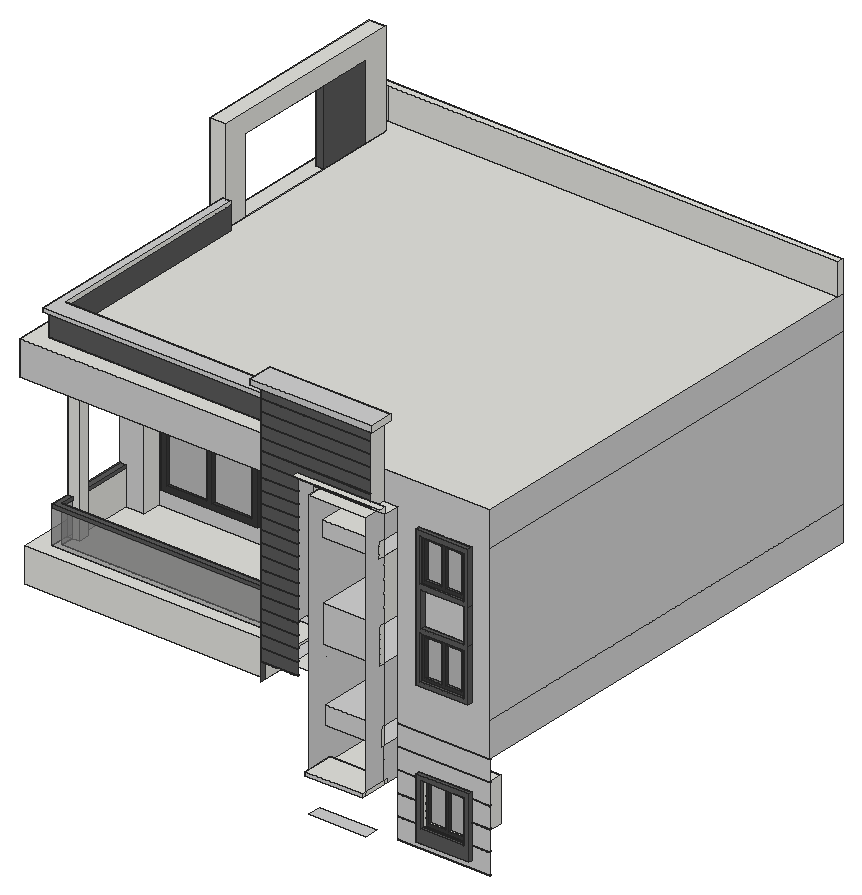
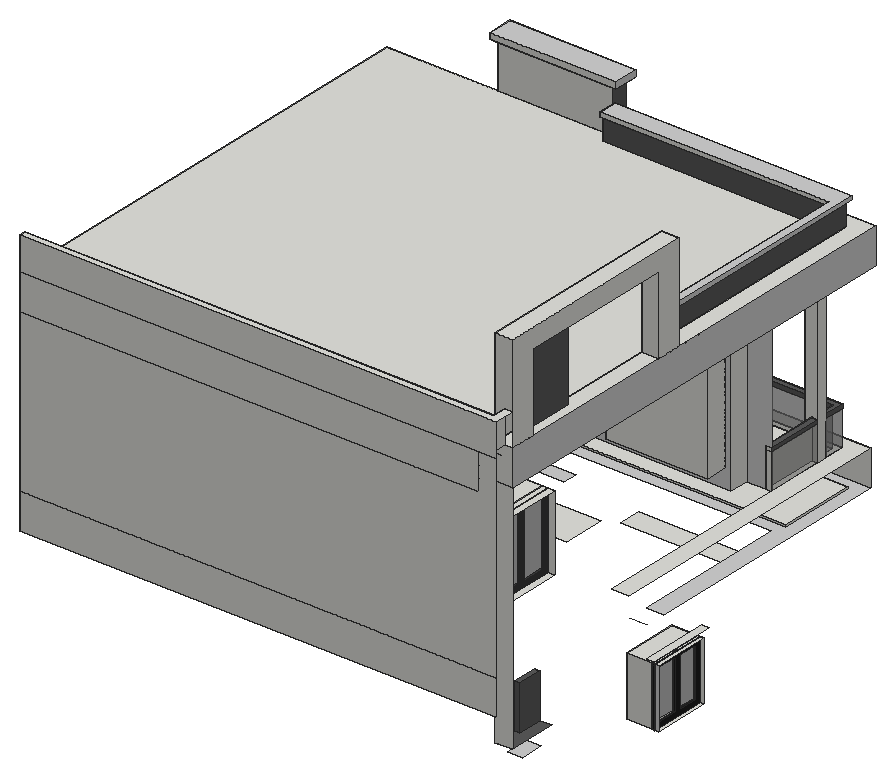
# SketchUp Ruby script. Lengths in inches.
U = 1.inch
M = Sketchup.active_model
def pt(a) = Geom::Point3d.new(a.map { |v| v * U })
def face(e, loops, mat)
  f = e.add_face(loops[0].map { |a| pt(a) })
  loops[1..].each { |l| e.add_face(l.map { |a| pt(a) }).erase! }
  f.material = f.back_material = mat if mat
  f
end
# faces: each face lists its corners as indices into pts; further lists are holes
def faces(e, pts, list, mat = nil) = list.each { |f| face(e, (f[0].is_a?(Array) ? f : [f]).map { |l| l.map { |i| pts[i] } }, mat) }
# xy, xz, yz: faces in a plane at the given z, y or x. An outline is a flat list of corners, or four numbers for a rectangle; further outlines are holes
def ring(l) = l.size == 4 ? [[l[0], l[1]], [l[2], l[1]], [l[2], l[3]], [l[0], l[3]]] : l.each_slice(2).to_a
def flat(e, list, mat, &to3) = list.each { |f| face(e, (f[0].is_a?(Array) ? f : [f]).map { |l| ring(l).map { |u, v| to3.(u, v) } }, mat) }
def xy(e, z, list, mat = nil) = flat(e, list, mat) { |x, y| [x, y, z] }
def xz(e, y, list, mat = nil) = flat(e, list, mat) { |x, z| [x, y, z] }
def yz(e, x, list, mat = nil) = flat(e, list, mat) { |y, z| [x, y, z] }
def lines(e, pts, list) = list.each { |a, b| e.add_line(pt(pts[a]), pt(pts[b])) }
# prism: a flat outline (further loops are holes) pulled along v
def prism(e, loops, v, mat = nil)
  f = face(e, loops, mat); d = Geom::Vector3d.new(v.map { |x| x * U })
  f.pushpull(f.normal.samedirection?(d) ? d.length : -d.length)
end
def box(e, o, s, mat = nil) = prism(e, [[o, [o[0] + s[0], o[1], o[2]], [o[0] + s[0], o[1] + s[1], o[2]], [o[0], o[1] + s[1], o[2]]]], [0, 0, s[2]], mat)
def at(x, y, z, deg = 0) = Geom::Transformation.translation(pt([x, y, z])) * Geom::Transformation.rotation(ORIGIN, Z_AXIS, deg.degrees)
def axes(o, x, y, z) = Geom::Transformation.new([*x, 0, *y, 0, *z, 0, *pt(o).to_a, 1])
def part(name) = M.definitions.add(name)
# library, detail: a bought-in or finely detailed component or shape, given as its bounding box
def library(name, o, s) = part(name).tap { |d| box(d.entities, o, s) }
def detail(e, o, s) = box(e.add_group.entities, o, s)
def put(e, d, t, mat = nil) = e.add_instance(d, t).tap { |i| i.material = mat if mat }
def group(e, t, mat = nil) = e.add_group.tap { |g| g.transformation = t; g.material = mat if mat }.entities
root = M.entities
M.materials.add("Generic").color = [90, 90, 90]
M.materials.add("Generic\#1").color = [208, 208, 208]
M.materials.add("[Color M06]").color = [86, 86, 86]
M.materials.add("[Color M07]").color = [58, 58, 58]
M.materials.add("[Color M08]").color = [30, 30, 30]
M.materials.add("[Mirror 01]").color = [185, 185, 185]
M.materials.add("[Translucent Glass Gray]").color = [128, 128, 128]
M.materials["[Translucent Glass Gray]"].alpha = 0.5
M.materials.add("[Wood Bamboo]").color = [177, 105, 43]
M.materials.add("[Wood Veneer 01]").color = [120, 70, 37]
c1 = part("Group\#1")
xy(c1.entities,0,[[0,0,47.4375,6]],"[Color M07]")
xy(c1.entities,3.58,[[3.58,0,21.93,3],[25.51,0,43.86,3]])
xy(c1.entities,43.86,[[3.58,0,21.93,3],[25.51,0,43.86,3]],"[Color M07]")
xy(c1.entities,47.4375,[[0,0,47.4375,6]],"[Color M07]")
xz(c1.entities,0,[[[0,0,47.4375,47.4375],[25.51,3.58,43.86,43.86],[3.58,3.58,21.93,43.86]]],"[Color M07]")
xz(c1.entities,3,[[3.58,3.58,21.93,43.86],[25.51,3.58,43.86,43.86]],"[Mirror 01]")
xz(c1.entities,6,[[0,0,47.4375,47.4375]],"[Mirror 01]")
yz(c1.entities,0,[[0,0,6,47.4375]],"[Color M07]")
yz(c1.entities,3.58,[[0,3.58,3,43.86]],"[Color M07]")
yz(c1.entities,21.93,[[0,3.58,3,43.86]],"[Color M07]")
yz(c1.entities,25.51,[[0,3.58,3,43.86]],"[Color M07]")
yz(c1.entities,43.86,[[0,3.58,3,43.86]],"[Color M06]")
yz(c1.entities,47.4375,[[0,0,6,47.4375]],"[Color M07]")
c2 = part("Group\#8")
xy(c2.entities,0,[[0,0,56.875,6.5]],"[Wood Veneer 01]")
xy(c2.entities,4.88,[[4.88,0,51.99,3.5]],"[Wood Veneer 01]")
xy(c2.entities,109.93,[[4.88,0,51.99,3.5]],"[Wood Veneer 01]")
xy(c2.entities,114.8125,[[0,0,56.875,6.5]],"[Wood Veneer 01]")
xz(c2.entities,0,[[[0,0,56.875,114.8125],[4.88,4.88,51.99,109.93]]],"[Wood Veneer 01]")
xz(c2.entities,0.5,[[8.38,56.46,8.6,56.49,8.8,56.57,8.97,56.7,9.1,56.88,9.1875,57.08,9.22,57.3,9.1875,57.51,9.1,57.71,8.97,57.89,8.8,58.02,8.6,58.1,8.38,58.13,8.16,58.1,7.96,58.02,7.79,57.89,7.66,57.71,7.57,57.51,7.54,57.3,7.57,57.08,7.66,56.88,7.79,56.7,7.96,56.57,8.16,56.49]],"[Wood Veneer 01]")
xz(c2.entities,3.5,[[8.38,56.46,8.16,56.49,7.96,56.57,7.79,56.7,7.66,56.88,7.57,57.08,7.54,57.3,7.57,57.51,7.66,57.71,7.79,57.89,7.96,58.02,8.16,58.1,8.38,58.13,8.6,58.1,8.8,58.02,8.97,57.89,9.1,57.71,9.1875,57.51,9.22,57.3,9.1875,57.08,9.1,56.88,8.97,56.7,8.8,56.57,8.6,56.49]])
xz(c2.entities,3.5,[[[4.88,4.88,51.99,109.93],[8.38,56.46,8.16,56.49,7.96,56.57,7.79,56.7,7.66,56.88,7.57,57.08,7.54,57.3,7.57,57.51,7.66,57.71,7.79,57.89,7.96,58.02,8.16,58.1,8.38,58.13,8.6,58.1,8.8,58.02,8.97,57.89,9.1,57.71,9.1875,57.51,9.22,57.3,9.1875,57.08,9.1,56.88,8.97,56.7,8.8,56.57,8.6,56.49]]],"[Wood Bamboo]")
xz(c2.entities,6.5,[[0,0,56.875,114.8125]],"[Wood Veneer 01]")
yz(c2.entities,0,[[0,0,6.5,114.8125]],"[Wood Veneer 01]")
yz(c2.entities,4.88,[[0,4.88,3.5,109.93]],"[Wood Veneer 01]")
yz(c2.entities,51.99,[[0,4.88,3.5,109.93]],"[Wood Veneer 01]")
yz(c2.entities,56.875,[[0,0,6.5,114.8125]],"[Wood Veneer 01]")
p = [[7.96,3.5,56.57],[8.16,3.5,56.49],[8.16,0.5,56.49],[7.96,0.5,56.57],[8.38,3.5,56.46],[8.38,0.5,56.46],
  [8.6,3.5,56.49],[8.6,0.5,56.49],[8.8,3.5,56.57],[8.8,0.5,56.57],[7.79,3.5,56.7],[7.79,0.5,56.7],
  [8.97,3.5,56.7],[8.97,0.5,56.7],[7.66,3.5,56.88],[7.66,0.5,56.88],[9.1,3.5,56.88],[9.1,0.5,56.88],
  [7.57,3.5,57.08],[7.57,0.5,57.08],[9.1875,3.5,57.08],[9.1875,0.5,57.08],[7.54,3.5,57.3],[7.54,0.5,57.3],
  [9.22,3.5,57.3],[9.22,0.5,57.3],[7.57,3.5,57.51],[7.57,0.5,57.51],[9.1875,3.5,57.51],[9.1875,0.5,57.51],
  [7.66,3.5,57.71],[7.66,0.5,57.71],[9.1,3.5,57.71],[9.1,0.5,57.71],[7.79,3.5,57.89],[7.79,0.5,57.89],
  [8.97,3.5,57.89],[8.97,0.5,57.89],[7.96,3.5,58.02],[7.96,0.5,58.02],[8.8,3.5,58.02],[8.8,0.5,58.02],
  [8.16,3.5,58.1],[8.16,0.5,58.1],[8.6,3.5,58.1],[8.6,0.5,58.1],[8.38,3.5,58.13],[8.38,0.5,58.13],
  [8.38,3.5,57.3],[8.38,0.5,57.3]]
faces(c2.entities,p,[[0,1,2,3],[1,4,5,2],[4,6,7,5],[6,8,9,7],[10,0,3,11],[8,12,13,9],[14,10,11,15],[12,16,17,13],
  [18,14,15,19],[16,20,21,17],[22,18,19,23],[20,24,25,21],[26,22,23,27],[24,28,29,25],[30,26,27,31],[28,32,33,29],
  [34,30,31,35],[32,36,37,33],[38,34,35,39],[36,40,41,37],[42,38,39,43],[40,44,45,41],[46,42,43,47],[44,46,47,45]],"[Wood Veneer 01]")
lines(c2.entities,p,[[48,49]])
c3 = part("Group\#7")
xy(c3.entities,0,[[0,0,106.25,6]],"[Color M07]")
xy(c3.entities,6.42,[[6.42,0,49.92,3],[56.33,0,99.83,3]],"[Color M07]")
xy(c3.entities,116.15,[[6.42,0,49.92,3],[56.33,0,99.83,3]],"[Color M07]")
xy(c3.entities,122.5625,[[0,0,106.25,6]],"[Color M07]")
xz(c3.entities,0,[[[0,0,106.25,122.5625],[56.33,6.42,99.83,116.15],[6.42,6.42,49.92,116.15]]],"[Color M07]")
xz(c3.entities,3,[[6.42,6.42,49.92,116.15],[56.33,6.42,99.83,116.15]],"[Mirror 01]")
xz(c3.entities,6,[[0,0,106.25,122.5625]],"[Mirror 01]")
yz(c3.entities,0,[[0,0,6,122.5625]],"[Color M07]")
yz(c3.entities,6.42,[[0,6.42,3,116.15]],"[Color M07]")
yz(c3.entities,49.92,[[0,6.42,3,116.15]],"[Color M07]")
yz(c3.entities,56.33,[[0,6.42,3,116.15]],"[Color M07]")
yz(c3.entities,99.83,[[0,6.42,3,116.15]],"[Color M07]")
yz(c3.entities,106.25,[[0,0,6,122.5625]],"[Color M07]")
xy(root,256.83,[[19.75,319.97,27.1875,379.02],[27.1875,319.97,53.1875,379.02]])
xy(root,259.46,[[406.8125,125.125,507.1875,126.125]])
xy(root,260.46,[[406.8125,125.125,507.1875,126.125]])
xy(root,267.4,[[328.9375,101.1875,391.1875,116.5]],"Generic\#1")
xy(root,267.49,[[429.86,121.125,487.29,125.125]],"Generic")
xy(root,281.55,[[434.86,125.125,482.3,170.75]])
xy(root,281.55,[[434.86,121.125,482.3,125.125]],"Generic")
xy(root,282.03,[[406.8125,125.125,429.86,126.125],[487.29,125.125,507.1875,126.125]])
xy(root,283.03,[[406.8125,125.125,429.86,126.125],[487.29,125.125,507.1875,126.125]])
xy(root,304.6,[[406.8125,125.125,429.86,126.125],[487.29,125.125,507.1875,126.125]])
xy(root,305.6,[[406.8125,125.125,429.86,126.125],[487.29,125.125,507.1875,126.125]])
xy(root,306.96,[[328.9375,101.1875,391.1875,130.25],[328.9375,130.25,391.1875,228.875]])
xy(root,306.96,[[328.9375,96.625,391.1875,101.1875]],"Generic\#1")
xy(root,311.15,[[328.9375,96.625,391.1875,130.25]])
xy(root,318.95,[[19.75,319.97,27.1875,379.02],[27.1875,319.97,53.1875,379.02]])
xy(root,320.02,[[9.25,545.63,25.375,569.56]],"Generic\#1")
xy(root,320.125,[[205.46,222.125,262.34,266.625]])
xy(root,325.58,[[19.75,313.34,27.1875,385.65]])
xy(root,327.17,[[406.8125,125.125,429.86,126.125],[487.29,125.125,507.1875,126.125]])
xy(root,328.17,[[406.8125,125.125,429.86,126.125],[487.29,125.125,507.1875,126.125]])
xy(root,328.98,[[434.86,125.125,482.3,170.75]])
xy(root,328.98,[[434.86,121.125,482.3,125.125]],"Generic")
xy(root,333.84,[[9.25,531.8125,21.875,531.8125,21.875,557.59,27.1875,557.59,27.1875,583.375,9.25,583.375]],"Generic")
xy(root,333.98,[[429.86,121.125,487.29,125.125]],"Generic")
xy(root,342.41,[[59.8,222.125,166.05,244.9375]])
xy(root,345.09,[[328.9375,123.1875,391.1875,228.875]],"Generic\#1")
xy(root,349.74,[[406.8125,125.125,507.1875,126.125]])
xy(root,350.74,[[406.8125,125.125,507.1875,126.125]])
xy(root,364.84,[[328.9375,123.1875,391.1875,228.875]],"Generic\#1")
xy(root,372.3125,[[406.8125,125.125,507.1875,126.125]])
xy(root,373.3125,[[406.8125,125.125,507.1875,126.125]])
xy(root,373.3125,[[[9.25,115,9.25,385.65,27.1875,385.65,27.1875,222.125,271.1875,222.125,271.1875,115],[22.25,128,258.19,209.13]]],"Generic\#1")
xy(root,375.25,[[22.25,128,258.19,209.13]])
xy(root,380.36,[[21.875,531.8125,27.1875,557.59]],"Generic")
xy(root,393.125,[[271.1875,108.0625,280.1875,109.1875],[280.1875,108.0625,283.1875,109.1875],[283.1875,108.0625,285.0625,109.1875],[285.0625,108.0625,288.0625,109.1875],[288.0625,108.0625,289.9375,109.1875],
  [289.9375,108.0625,292.9375,109.1875],[292.9375,108.0625,294.8125,109.1875],[294.8125,108.0625,297.8125,109.1875],[297.8125,108.0625,299.6875,109.1875],[299.6875,108.0625,302.6875,109.1875],
  [302.6875,108.0625,304.5625,109.1875],[304.5625,108.0625,307.5625,109.1875],[307.5625,108.0625,311.625,109.1875]])
xy(root,394.125,[[271.1875,108.0625,311.625,109.1875]])
xy(root,405.9375,[[271.1875,108.0625,311.625,109.1875]])
xy(root,406.9375,[[271.1875,108.0625,311.625,109.1875]])
xy(root,410.625,[[9.25,115,271.1875,115,271.1875,129.3125,27.1875,129.3125,27.1875,430.9,9.25,430.9],[27.1875,129.3125,27.1875,150.52,32.5,150.52,32.5,135.5625,271.1875,135.5625,271.1875,129.3125],[32.5,135.5625,32.5,150.52,40.39,150.52,40.39,162.02,33.3125,162.02,33.3125,222.125,53.1875,222.125,53.1875,242.1875,271.1875,242.1875,271.1875,135.5625],[27.1875,150.52,40.39,162.02],[27.1875,162.02,33.3125,222.125]])
xy(root,415.3125,[[205.46,242.1875,262.34,283.1875]])
xy(root,418.75,[[271.1875,108.0625,311.625,109.1875]])
xy(root,419.75,[[271.1875,108.0625,311.625,109.1875]])
xy(root,421.02,[[430.14,120.125,487.01,125.125]],"Generic")
xy(root,425.4,[[328.9375,120.3125,391.1875,228.875]],"Generic\#1")
xy(root,425.73,[[434.86,125.125,482.3,177.0625]])
xy(root,425.73,[[434.86,120.125,482.3,125.125]],"Generic")
xy(root,429.84,[[59.8,242.1875,166.05,265]])
xy(root,431.5625,[[271.1875,108.0625,311.625,109.1875]])
xy(root,432.5625,[[271.1875,108.0625,311.625,109.1875]])
xy(root,444.375,[[271.1875,108.0625,311.625,109.1875]])
xy(root,445.375,[[271.1875,108.0625,311.625,109.1875]])
xy(root,447.5,[[27.1875,129.3125,27.1875,150.52,32.5,150.52,32.5,135.5625,271.1875,135.5625,271.1875,129.3125],[27.1875,162.02,33.3125,222.125]])
xy(root,451.5,[[27.1875,129.3125,271.1875,129.3125,271.1875,135.5625,32.5,135.5625,32.5,150.52,27.1875,150.52],[27.1875,162.02,33.3125,222.125]],"Generic")
xy(root,456.26,[[27.1875,505.08,76.625,574.96]])
xy(root,457.1875,[[271.1875,108.0625,311.625,109.1875]])
xy(root,458.1875,[[271.1875,108.0625,311.625,109.1875]])
xy(root,464.84,[[328.9375,120.3125,391.1875,228.875]],"Generic\#1")
xy(root,470,[[271.1875,108.0625,311.625,109.1875]])
xy(root,471,[[271.1875,108.0625,311.625,109.1875]])
xy(root,473.17,[[434.86,125.125,482.3,177.0625]])
xy(root,473.17,[[434.86,120.125,482.3,125.125]],"Generic")
xy(root,477.89,[[435.91,120.125,482.26,125.125]],"Generic")
xy(root,482.8125,[[271.1875,108.0625,311.625,109.1875]])
xy(root,483.8125,[[271.1875,108.0625,311.625,109.1875]])
xy(root,495.625,[[271.1875,108.0625,311.625,109.1875]])
xy(root,496.625,[[271.1875,108.0625,311.625,109.1875]])
xy(root,508.4375,[[271.1875,108.0625,311.625,109.1875]])
xy(root,509.4375,[[271.1875,108.0625,311.625,109.1875]])
xy(root,515.77,[[435.91,120.125,482.26,125.125]],"Generic")
xy(root,520.48,[[434.86,125.125,482.3,177.0625]])
xy(root,520.48,[[434.86,120.125,482.3,125.125]],"Generic")
xy(root,521.25,[[271.1875,108.0625,311.625,109.1875]])
xy(root,522.25,[[271.1875,108.0625,311.625,109.1875]])
xy(root,529.9,[[328.9375,119.4375,391.1875,228.875]],"Generic\#1")
xy(root,530.125,[[205.46,242.1875,262.34,283.1875]])
xy(root,534.0625,[[271.1875,108.0625,311.625,109.1875]])
xy(root,535.0625,[[271.1875,108.0625,311.625,109.1875]])
xy(root,535.64,[[27.1875,505.08,76.625,574.96]])
xy(root,546.71,[[328.9375,119.4375,391.1875,228.875]])
xy(root,546.875,[[271.1875,108.0625,311.625,109.1875]])
xy(root,547.875,[[271.1875,108.0625,311.625,109.1875]])
xy(root,552.41,[[59.8,242.1875,166.05,265]])
xy(root,559.6875,[[271.1875,108.0625,311.625,109.1875]])
xy(root,560.6875,[[271.1875,108.0625,311.625,109.1875]])
xy(root,567.92,[[434.86,125.125,482.3,177.0625]])
xy(root,567.92,[[434.86,120.125,482.3,125.125]],"Generic")
xy(root,572.5,[[271.1875,108.0625,311.625,109.1875]])
xy(root,572.64,[[430.14,120.125,487.01,125.125]],"Generic")
xy(root,573.5,[[271.1875,108.0625,311.625,109.1875]])
xy(root,578.625,[[328.9375,101.1875,391.1875,228.875],[271.1875,125.125,319.1875,137]])
xy(root,578.625,[[9.25,108.0625,9.25,583.375,27.1875,583.375,27.1875,125.125,271.1875,125.125,271.1875,108.0625],[[27.1875,125.125,27.1875,150.52,40.39,150.52,40.39,162.02,27.1875,162.02,27.1875,222.125,53.1875,222.125,53.1875,242.1875,271.1875,242.1875,271.1875,125.125],[55.86,140.6,255.72,226.72]]],"Generic\#1")
xy(root,580.9375,[[55.86,140.6,255.72,226.72]])
xy(root,584.3125,[[328.9375,108.0625,391.1875,125.125],[391.1875,108.0625,406.8125,125.125]])
xy(root,585.3125,[[271.1875,108.0625,311.625,109.1875]])
xy(root,586.3125,[[271.1875,108.0625,311.625,109.1875]])
xy(root,591.5625,[[311.625,101.1875,406.8125,108.0625]])
xy(root,598.125,[[271.1875,108.0625,391.1875,109.1875]])
xy(root,599.125,[[271.1875,108.0625,391.1875,109.1875]])
xy(root,610.9375,[[271.1875,108.0625,391.1875,109.1875]])
xy(root,611.9375,[[271.1875,108.0625,391.1875,109.1875]])
xy(root,615.9375,[[9.25,108.0625,271.1875,108.0625,271.1875,125.125,27.1875,125.125,27.1875,366.125,9.25,366.125],[271.1875,125.125,507.1875,125.125,507.1875,598,17.4375,598,17.4375,583.375,27.1875,583.375,27.1875,366.125,32.375,366.125,32.375,137.4375,271.1875,137.4375],[9.25,366.125,27.1875,392.17],[9.25,392.17,27.1875,392.17,27.1875,498.875,18.5,498.875,18.5,556.25,9.25,556.25],[9.25,556.25,27.1875,583.375]])
xy(root,623.75,[[271.1875,108.0625,391.1875,109.1875]])
xy(root,624.75,[[271.1875,108.0625,391.1875,109.1875]])
xy(root,636.5625,[[271.1875,108.0625,391.1875,109.1875]])
xy(root,637.5625,[[271.1875,108.0625,391.1875,109.1875]])
xy(root,640.625,[[23.4375,121.375,271.1875,125.125],[23.4375,125.125,27.1875,366.125],[27.1875,125.125,27.1875,366.125,32.375,366.125,32.375,137.4375,271.1875,137.4375,271.1875,125.125],[32.375,137.4375,271.1875,141.1875]])
xy(root,645,[[23.4375,121.375,271.1875,121.375,271.1875,141.1875,32.375,141.1875,32.375,366.125,23.4375,366.125]],"Generic\#1")
xy(root,649.375,[[271.1875,108.0625,391.1875,109.1875]])
xy(root,650.375,[[271.1875,108.0625,391.1875,109.1875]])
xy(root,650.4375,[[9.25,583.375,17.4375,583.375,17.4375,598,507.1875,598,507.1875,605.125,9.25,605.125]])
xy(root,663.125,[[264.9375,101.8125,397.125,108.0625],[264.9375,108.0625,271.1875,128.125],[271.1875,108.0625,391.1875,125.125],[391.1875,108.0625,397.125,128.125],[271.1875,125.125,391.1875,128.125]])
xy(root,669.5,[[264.9375,101.8125,397.125,128.125]],"Generic\#1")
xy(root,697.0625,[[9.25,392.17,9.25,556.25,18.5,556.25,18.5,498.875,27.1875,498.875,27.1875,392.17]])
xy(root,717.9375,[[9.25,366.125,27.1875,583.375]])
xz(root,96.625,[[328.9375,306.96,391.1875,311.15]],"Generic\#1")
xz(root,101.8125,[[264.9375,663.125,397.125,669.5]],"Generic\#1")
xz(root,108.0625,[[328.9375,584.3125,391.1875,585.3125],[391.1875,584.3125,406.8125,591.5625],[311.625,585.3125,328.9375,586.3125],[328.9375,585.3125,391.1875,586.3125],[328.9375,586.3125,391.1875,591.5625]])
xz(root,108.0625,[[271.1875,394.125,311.625,405.9375],[271.1875,406.9375,311.625,418.75],[271.1875,419.75,311.625,431.5625],[271.1875,432.5625,311.625,444.375],[271.1875,445.375,311.625,457.1875],
  [271.1875,458.1875,311.625,470],[271.1875,471,311.625,482.8125],[271.1875,483.8125,311.625,495.625],[271.1875,496.625,311.625,508.4375],[271.1875,509.4375,311.625,521.25],
  [271.1875,522.25,311.625,534.0625],[271.1875,535.0625,311.625,546.875],[271.1875,547.875,311.625,559.6875],[271.1875,560.6875,311.625,572.5],[271.1875,573.5,311.625,585.3125],
  [271.1875,586.3125,311.625,586.3125,311.625,591.5625,391.1875,591.5625,391.1875,598.125,271.1875,598.125],[271.1875,599.125,391.1875,610.9375],[271.1875,611.9375,391.1875,623.75],[271.1875,624.75,391.1875,636.5625],[271.1875,637.5625,391.1875,649.375],
  [271.1875,650.375,391.1875,663.125]],"Generic")
xz(root,108.0625,[[9.25,578.625,271.1875,615.9375]],"Generic\#1")
xz(root,109.1875,[[271.1875,393.125,311.625,394.125],[271.1875,405.9375,311.625,406.9375],[271.1875,418.75,311.625,419.75],[271.1875,431.5625,311.625,432.5625],[271.1875,444.375,311.625,445.375],
  [271.1875,457.1875,311.625,458.1875],[271.1875,470,311.625,471],[271.1875,482.8125,311.625,483.8125],[271.1875,495.625,311.625,496.625],[271.1875,508.4375,311.625,509.4375],
  [271.1875,521.25,311.625,522.25],[271.1875,534.0625,311.625,535.0625],[271.1875,546.875,311.625,547.875],[271.1875,559.6875,311.625,560.6875],[271.1875,572.5,311.625,573.5],
  [271.1875,585.3125,311.625,586.3125],[271.1875,598.125,391.1875,599.125],[271.1875,610.9375,391.1875,611.9375],[271.1875,623.75,391.1875,624.75],[271.1875,636.5625,391.1875,637.5625],
  [271.1875,649.375,391.1875,650.375]])
xz(root,115,[[9.25,373.3125,271.1875,410.625]])
xz(root,119.4375,[[328.9375,529.9,391.1875,546.71]],"Generic\#1")
xz(root,120.125,[[[430.14,421.02,487.01,572.64],[434.86,425.73,482.3,473.17],[434.86,520.48,482.3,567.92],[435.91,477.89,482.26,515.77]]],"Generic")
xz(root,120.3125,[[328.9375,425.4,391.1875,464.84]],"Generic\#1")
xz(root,121.125,[[[429.86,267.49,487.29,333.98],[434.86,281.55,482.3,328.98]]],"Generic")
xz(root,121.375,[[23.4375,640.625,271.1875,645]],"Generic\#1")
xz(root,123.1875,[[328.9375,345.09,391.1875,364.84]],"Generic\#1")
xz(root,125.125,[[429.86,267.49,429.86,282.03,434.86,282.03,434.86,281.55,482.3,281.55,482.3,282.03,487.29,282.03,487.29,267.49],[429.86,282.03,434.86,283.03],[482.3,282.03,487.29,283.03],[429.86,283.03,434.86,304.6],[482.3,283.03,487.29,304.6],
  [429.86,304.6,434.86,305.6],[482.3,304.6,487.29,305.6],[429.86,305.6,434.86,327.17],[482.3,305.6,487.29,327.17],[429.86,327.17,434.86,328.17],
  [482.3,327.17,487.29,328.17],[429.86,328.17,429.86,333.98,487.29,333.98,487.29,328.17,482.3,328.17,482.3,328.98,434.86,328.98,434.86,328.17],[[430.14,421.02,487.01,477.89],[434.86,425.73,482.3,473.17]],[[430.14,477.89,430.14,572.64,487.01,572.64,487.01,515.77,435.91,515.77,435.91,477.89],[434.86,520.48,482.3,567.92]],[482.26,477.89,487.01,515.77],
  [27.1875,578.625,271.1875,615.9375],[271.1875,578.625,328.9375,578.625,328.9375,584.3125,391.1875,584.3125,391.1875,615.9375,271.1875,615.9375],[271.1875,615.9375,391.1875,663.125]])
xz(root,125.125,[[27.1875,615.9375,271.1875,640.625]],"Generic")
xz(root,125.125,[[406.8125,260.46,507.1875,260.46,507.1875,282.03,487.29,282.03,487.29,267.49,429.86,267.49,429.86,282.03,406.8125,282.03],[406.8125,283.03,429.86,304.6],[487.29,283.03,507.1875,304.6],[406.8125,305.6,429.86,327.17],[487.29,305.6,507.1875,327.17],
  [406.8125,328.17,429.86,328.17,429.86,333.98,487.29,333.98,487.29,328.17,507.1875,328.17,507.1875,349.74,406.8125,349.74],[406.8125,350.74,507.1875,372.3125],[[406.8125,373.3125,507.1875,373.3125,507.1875,615.9375,391.1875,615.9375,391.1875,584.3125,406.8125,584.3125],[430.14,421.02,487.01,572.64]],[435.91,477.89,482.26,515.77]],"Generic\#1")
xz(root,126.125,[[406.8125,259.46,507.1875,260.46],[406.8125,282.03,429.86,283.03],[487.29,282.03,507.1875,283.03],[406.8125,304.6,429.86,305.6],[487.29,304.6,507.1875,305.6],
  [406.8125,327.17,429.86,328.17],[487.29,327.17,507.1875,328.17],[406.8125,349.74,507.1875,350.74],[406.8125,372.3125,507.1875,373.3125]])
xz(root,128,[[22.25,373.3125,258.19,375.25]])
xz(root,128.125,[[264.9375,663.125,397.125,669.5]])
xz(root,129.3125,[[27.1875,447.5,271.1875,451.5]],"Generic")
xz(root,129.3125,[[27.1875,410.625,271.1875,447.5]],"[Translucent Glass Gray]")
xz(root,130.25,[[328.9375,306.96,391.1875,311.15]])
xz(root,135.5625,[[32.5,447.5,271.1875,451.5]],"Generic")
xz(root,135.5625,[[32.5,410.625,271.1875,447.5]],"[Translucent Glass Gray]")
xz(root,137.4375,[[32.375,615.9375,271.1875,640.625]],"Generic")
xz(root,140.6,[[55.86,578.625,255.72,580.9375]])
xz(root,141.1875,[[32.375,640.625,271.1875,645]])
xz(root,150.52,[[32.5,410.625,40.39,410.625,40.39,578.625,27.1875,578.625,27.1875,451.5,32.5,451.5]])
xz(root,162.02,[[27.1875,410.625,33.3125,447.5],[33.3125,410.625,33.3125,451.5,27.1875,451.5,27.1875,578.625,40.39,578.625,40.39,410.625],[27.1875,447.5,33.3125,451.5]])
xz(root,170.75,[[434.86,281.55,482.3,328.98]])
xz(root,177.0625,[[434.86,425.73,482.3,473.17],[434.86,520.48,482.3,567.92]])
xz(root,209.13,[[22.25,373.3125,258.19,375.25]])
xz(root,222.125,[[27.1875,410.625,33.3125,447.5],[27.1875,447.5,33.3125,451.5]])
xz(root,222.125,[[33.3125,410.625,53.1875,410.625,53.1875,578.625,27.1875,578.625,27.1875,451.5,33.3125,451.5]],"Generic\#1")
xz(root,226.72,[[55.86,578.625,255.72,580.9375]])
xz(root,228.875,[[328.9375,306.96,391.1875,345.09],[328.9375,364.84,391.1875,425.4],[328.9375,464.84,391.1875,529.9],[328.9375,546.71,391.1875,578.625]],"Generic\#1")
xz(root,242.1875,[[[53.1875,410.625,271.1875,578.625],[59.8,429.84,166.05,552.41],[205.46,415.3125,262.34,530.125]]],"Generic\#1")
xz(root,265,[[59.8,429.84,166.05,552.41]])
xz(root,283.1875,[[205.46,415.3125,262.34,530.125]])
xz(root,319.97,[[19.75,256.83,27.1875,318.95],[27.1875,256.83,53.1875,318.95]])
xz(root,366.125,[[9.25,615.9375,27.1875,615.9375,27.1875,640.625,23.4375,640.625,23.4375,645,27.1875,645,27.1875,717.9375,9.25,717.9375],[27.1875,615.9375,32.375,640.625],[23.4375,640.625,27.1875,645],[27.1875,640.625,32.375,645]])
xz(root,379.02,[[27.1875,256.83,53.1875,318.95]])
xz(root,379.02,[[19.75,256.83,27.1875,318.95]],"Generic\#1")
xz(root,392.17,[[9.25,615.9375,27.1875,697.0625]])
xz(root,498.875,[[18.5,615.9375,27.1875,697.0625]],"Generic")
xz(root,505.08,[[27.1875,456.26,76.625,535.64]])
xz(root,531.8125,[[21.875,333.84,27.1875,380.36]],"Generic")
xz(root,556.25,[[9.25,615.9375,18.5,697.0625],[18.5,615.9375,27.1875,697.0625]])
xz(root,557.59,[[21.875,333.84,27.1875,380.36]],"Generic")
xz(root,574.96,[[27.1875,456.26,76.625,535.64]])
xz(root,583.375,[[9.25,333.84,27.1875,578.625],[9.25,578.625,27.1875,615.9375],[17.4375,615.9375,17.4375,650.4375,9.25,650.4375,9.25,717.9375,27.1875,717.9375,27.1875,615.9375]])
xz(root,598,[[17.4375,615.9375,507.1875,650.4375]])
xz(root,605.125,[[9.25,373.3125,507.1875,410.625],[9.25,410.625,9.25,615.9375,27.1875,615.9375,27.1875,578.625,507.1875,578.625,507.1875,410.625],[27.1875,578.625,507.1875,615.9375],[9.25,615.9375,507.1875,650.4375]])
yz(root,9.25,[[366.125,615.9375,366.125,717.9375,583.375,717.9375,583.375,615.9375,556.25,615.9375,556.25,697.0625,392.17,697.0625,392.17,615.9375]])
yz(root,9.25,[[108.0625,578.625,583.375,615.9375]],"Generic\#1")
yz(root,17.4375,[[583.375,615.9375,598,650.4375]])
yz(root,18.5,[[498.875,615.9375,556.25,697.0625]],"Generic")
yz(root,21.875,[[531.8125,333.84,557.59,380.36]],"Generic")
yz(root,22.25,[[128,373.3125,209.13,375.25]])
yz(root,23.4375,[[121.375,640.625,366.125,645]],"Generic\#1")
yz(root,27.1875,[[150.52,410.625,162.02,578.625],[125.125,578.625,583.375,615.9375],[366.125,615.9375,392.17,615.9375,392.17,697.0625,556.25,697.0625,556.25,615.9375,583.375,615.9375,583.375,717.9375,366.125,717.9375]])
yz(root,27.1875,[[129.3125,447.5,150.52,451.5],[162.02,447.5,222.125,451.5],[125.125,615.9375,366.125,640.625],[498.875,615.9375,556.25,697.0625]],"Generic")
yz(root,27.1875,[[129.3125,410.625,150.52,447.5],[162.02,410.625,222.125,447.5]],"[Translucent Glass Gray]")
yz(root,32.375,[[141.1875,640.625,366.125,645]])
yz(root,32.375,[[137.4375,615.9375,366.125,640.625]],"Generic")
yz(root,32.5,[[135.5625,447.5,150.52,451.5]],"Generic")
yz(root,32.5,[[135.5625,410.625,150.52,447.5]],"[Translucent Glass Gray]")
yz(root,33.3125,[[162.02,410.625,222.125,447.5]])
yz(root,33.3125,[[162.02,447.5,222.125,451.5]],"Generic")
yz(root,40.39,[[150.52,410.625,162.02,578.625]])
yz(root,53.1875,[[319.97,256.83,379.02,318.95],[222.125,410.625,242.1875,578.625]])
yz(root,55.86,[[140.6,578.625,177.49,580.9375],[177.49,578.625,206.65,580.9375],[206.65,578.625,226.72,580.9375]])
yz(root,59.8,[[242.1875,429.84,265,552.41]])
yz(root,76.625,[[505.08,456.26,574.96,535.64]])
yz(root,166.05,[[242.1875,429.84,265,552.41]])
yz(root,205.46,[[242.1875,415.3125,283.1875,530.125]])
yz(root,255.72,[[140.6,578.625,226.72,580.9375]])
yz(root,258.19,[[128,373.3125,137,375.25],[137,373.3125,209.13,375.25]])
yz(root,262.34,[[242.1875,415.3125,283.1875,530.125]])
yz(root,264.9375,[[101.8125,663.125,128.125,669.5]],"Generic\#1")
yz(root,271.1875,[[115,373.3125,137,410.625],[129.3125,410.625,135.5625,447.5],[129.3125,447.5,135.5625,451.5],[108.0625,578.625,108.0625,585.3125,109.1875,585.3125,109.1875,586.3125,108.0625,586.3125,108.0625,598.125,109.1875,598.125,109.1875,599.125,108.0625,599.125,108.0625,610.9375,109.1875,610.9375,109.1875,611.9375,108.0625,611.9375,108.0625,615.9375,125.125,615.9375,125.125,578.625],[108.0625,585.3125,109.1875,586.3125],
  [108.0625,598.125,109.1875,599.125],[108.0625,610.9375,109.1875,611.9375],[125.125,615.9375,137.4375,640.625],[121.375,640.625,125.125,645],[125.125,640.625,141.1875,645]])
yz(root,271.1875,[[108.0625,373.3125,108.0625,393.125,109.1875,393.125,109.1875,394.125,108.0625,394.125,108.0625,405.9375,109.1875,405.9375,109.1875,406.9375,108.0625,406.9375,108.0625,410.625,115,410.625,115,373.3125],[108.0625,410.625,108.0625,418.75,109.1875,418.75,109.1875,419.75,108.0625,419.75,108.0625,431.5625,109.1875,431.5625,109.1875,432.5625,108.0625,432.5625,108.0625,444.375,109.1875,444.375,109.1875,445.375,108.0625,445.375,108.0625,457.1875,109.1875,457.1875,109.1875,458.1875,108.0625,458.1875,108.0625,470,109.1875,470,109.1875,471,108.0625,471,108.0625,482.8125,109.1875,482.8125,109.1875,483.8125,108.0625,483.8125,108.0625,495.625,109.1875,495.625,109.1875,496.625,108.0625,496.625,108.0625,508.4375,109.1875,508.4375,109.1875,509.4375,108.0625,509.4375,108.0625,521.25,109.1875,521.25,109.1875,522.25,108.0625,522.25,108.0625,534.0625,109.1875,534.0625,109.1875,535.0625,108.0625,535.0625,108.0625,546.875,109.1875,546.875,109.1875,547.875,108.0625,547.875,108.0625,559.6875,109.1875,559.6875,109.1875,560.6875,108.0625,560.6875,108.0625,572.5,109.1875,572.5,109.1875,573.5,108.0625,573.5,108.0625,578.625,137,578.625,137,410.625,135.5625,410.625,135.5625,451.5,129.3125,451.5,129.3125,410.625],[108.0625,615.9375,108.0625,623.75,109.1875,623.75,109.1875,624.75,108.0625,624.75,108.0625,636.5625,109.1875,636.5625,109.1875,637.5625,108.0625,637.5625,108.0625,649.375,109.1875,649.375,109.1875,650.375,108.0625,650.375,108.0625,663.125,125.125,663.125,125.125,645,121.375,645,121.375,640.625,125.125,640.625,125.125,615.9375]],"Generic")
yz(root,271.1875,[[137,410.625,242.1875,578.625]],"Generic\#1")
yz(root,311.625,[[108.0625,585.3125,109.1875,586.3125]])
yz(root,319.1875,[[125.125,373.3125,137,410.625],[125.125,410.625,137,578.625]])
yz(root,328.9375,[[96.625,306.96,101.1875,311.15],[101.1875,306.96,125.125,311.15],[125.125,306.96,130.25,311.15],[108.0625,578.625,125.125,584.3125]])
yz(root,328.9375,[[130.25,306.96,228.875,306.96,228.875,345.09,123.1875,345.09,123.1875,364.84,228.875,364.84,228.875,425.4,120.3125,425.4,120.3125,464.84,228.875,464.84,228.875,529.9,119.4375,529.9,119.4375,546.71,228.875,546.71,228.875,578.625,101.1875,578.625,101.1875,311.15,130.25,311.15]],"Generic\#1")
yz(root,391.1875,[[96.625,306.96,101.1875,311.15],[101.1875,306.96,125.125,311.15],[125.125,306.96,130.25,311.15],[123.1875,345.09,125.125,364.84],[120.3125,425.4,125.125,464.84],
  [125.125,464.84,228.875,529.9],[119.4375,529.9,125.125,546.71],[108.0625,584.3125,125.125,584.3125,125.125,663.125,108.0625,663.125,108.0625,650.375,109.1875,650.375,109.1875,649.375,108.0625,649.375,108.0625,637.5625,109.1875,637.5625,109.1875,636.5625,108.0625,636.5625,108.0625,624.75,109.1875,624.75,109.1875,623.75,108.0625,623.75,108.0625,611.9375,109.1875,611.9375,109.1875,610.9375,108.0625,610.9375,108.0625,599.125,109.1875,599.125,109.1875,598.125,108.0625,598.125]])
yz(root,391.1875,[[130.25,306.96,130.25,311.15,125.125,311.15,125.125,345.09,228.875,345.09,228.875,306.96],[101.1875,311.15,101.1875,578.625,125.125,578.625,125.125,546.71,119.4375,546.71,119.4375,529.9,125.125,529.9,125.125,464.84,120.3125,464.84,120.3125,425.4,125.125,425.4,125.125,364.84,123.1875,364.84,123.1875,345.09,125.125,345.09,125.125,311.15],[125.125,364.84,228.875,425.4],[125.125,546.71,228.875,578.625]],"Generic\#1")
yz(root,397.125,[[101.8125,663.125,128.125,669.5]])
yz(root,406.8125,[[125.125,259.46,126.125,260.46],[125.125,282.03,126.125,283.03],[125.125,304.6,126.125,305.6],[125.125,327.17,126.125,328.17],[125.125,349.74,126.125,350.74],
  [125.125,372.3125,126.125,373.3125]])
yz(root,429.86,[[125.125,282.03,126.125,283.03],[125.125,304.6,126.125,305.6],[125.125,327.17,126.125,328.17]])
yz(root,429.86,[[121.125,267.49,125.125,333.98]],"Generic")
yz(root,430.14,[[120.125,421.02,125.125,477.89],[120.125,477.89,125.125,572.64]],"Generic")
yz(root,434.86,[[125.125,281.55,170.75,328.98],[125.125,425.73,177.0625,473.17],[125.125,520.48,177.0625,567.92]])
yz(root,434.86,[[121.125,281.55,125.125,328.98],[120.125,425.73,125.125,473.17],[120.125,520.48,125.125,567.92]],"Generic")
yz(root,435.91,[[120.125,477.89,125.125,515.77]],"Generic")
yz(root,482.26,[[120.125,477.89,125.125,515.77]],"Generic")
yz(root,482.3,[[125.125,281.55,170.75,328.98],[125.125,425.73,177.0625,473.17],[125.125,520.48,177.0625,567.92]])
yz(root,482.3,[[121.125,281.55,125.125,328.98],[120.125,425.73,125.125,473.17],[120.125,520.48,125.125,567.92]],"Generic")
yz(root,487.01,[[120.125,421.02,125.125,477.89],[120.125,477.89,125.125,515.77],[120.125,515.77,125.125,572.64]],"Generic")
yz(root,487.29,[[125.125,282.03,126.125,283.03],[125.125,304.6,126.125,305.6],[125.125,327.17,126.125,328.17]])
yz(root,487.29,[[121.125,267.49,125.125,333.98]],"Generic")
yz(root,507.1875,[[598,615.9375,605.125,650.4375]])
yz(root,507.1875,[[125.125,373.3125,605.125,410.625],[125.125,410.625,605.125,578.625],[125.125,578.625,605.125,615.9375]],"Generic\#1")
p = [[319.1875,125.125,410.625],[328.9375,125.125,410.625],[27.1875,407.53,373.3125],[9.25,407.53,373.3125],[17.4375,598,615.9375],[9.25,598,615.9375]]
lines(root,p,[[0,1],[2,3],[4,5]])
g1 = group(root,at(23.47,319.97,256.83))
xy(g1,0,[[0,0,3,59.05]],"[Color M08]")
xy(g1,5.21,[[0,5.21,3,26.92],[0,32.13,3,53.84]],"[Color M08]")
xy(g1,56.91,[[0,5.21,3,26.92],[0,32.13,3,53.84]],"[Color M08]")
xy(g1,62.12,[[0,0,3,59.05]],"[Color M08]")
xz(g1,0,[[0,0,3,62.12]],"[Color M08]")
xz(g1,5.21,[[0,5.21,3,56.91]],"[Color M08]")
xz(g1,26.92,[[0,5.21,3,56.91]],"[Color M08]")
xz(g1,32.13,[[0,5.21,3,56.91]],"[Color M08]")
xz(g1,53.84,[[0,5.21,3,56.91]],"[Color M08]")
xz(g1,59.05,[[0,0,3,62.12]],"[Color M08]")
yz(g1,0,[[[0,0,59.05,62.12],[32.13,5.21,53.84,56.91],[5.21,5.21,26.92,56.91]]],"[Color M08]")
yz(g1,3,[[[0,0,59.05,62.12],[32.13,5.21,53.84,56.91],[5.21,5.21,26.92,56.91]]])
yz(g1,3,[[5.21,5.21,26.92,56.91],[32.13,5.21,53.84,56.91]],"[Mirror 01]")
put(root,c1,at(434.86,127.9375,281.55))
put(root,c2,at(205.46,242.1875,415.3125))
put(root,c1,at(434.86,123.125,425.73),"Generic")
put(root,c3,at(59.8,236.1875,429.84))
g2 = group(root,at(34.5625,505.08,456.26))
xy(g2,0,[[0,0,6,69.875]],"[Color M07]")
xy(g2,5.4,[[0,5.4,3,32.24],[0,37.64,3,64.48]],"[Color M07]")
xy(g2,73.98,[[0,5.4,3,32.24],[0,37.64,3,64.48]],"[Color M07]")
xy(g2,79.375,[[0,0,6,69.875]],"[Color M07]")
xz(g2,0,[[0,0,6,79.375]])
xz(g2,5.4,[[0,5.4,3,73.98]],"[Color M07]")
xz(g2,32.24,[[0,5.4,3,73.98]])
xz(g2,37.64,[[0,5.4,3,73.98]],"[Color M07]")
xz(g2,64.48,[[0,5.4,3,73.98]],"[Color M07]")
xz(g2,69.875,[[0,0,6,79.375]],"[Color M07]")
yz(g2,0,[[[0,0,69.875,79.375],[37.64,5.4,64.48,73.98],[5.4,5.4,32.24,73.98]]],"[Color M07]")
yz(g2,3,[[5.4,5.4,32.24,73.98],[37.64,5.4,64.48,73.98]],"[Mirror 01]")
yz(g2,6,[[0,0,69.875,79.375]],"[Mirror 01]")
put(root,c1,at(434.86,123.125,520.48),"Generic")
